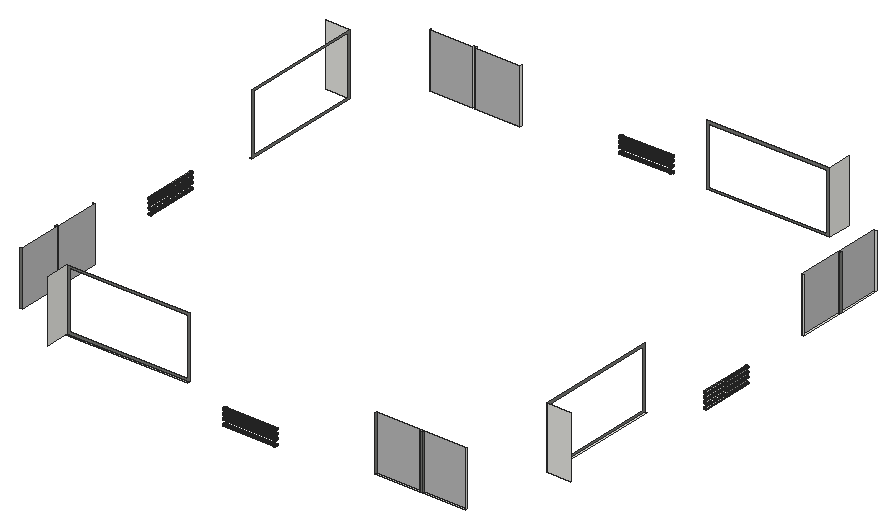
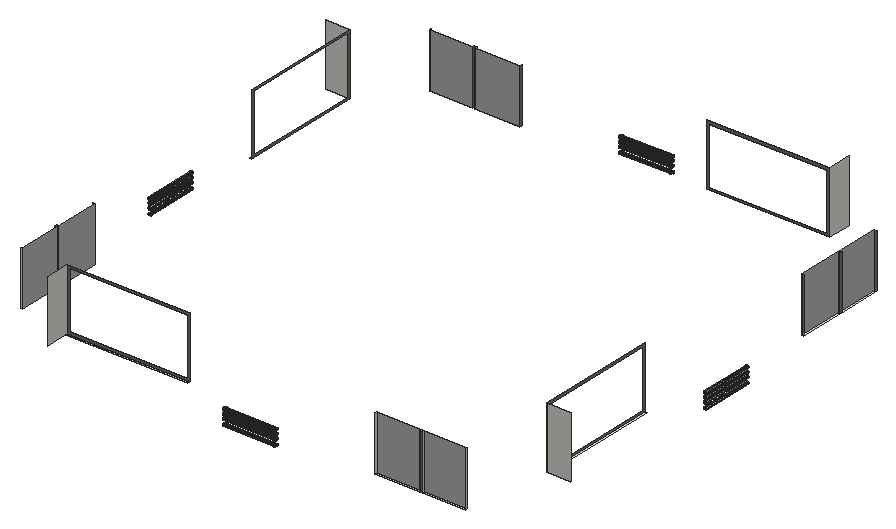
# SketchUp Ruby script. Lengths in inches.
U = 1.inch
M = Sketchup.active_model
def pt(a) = Geom::Point3d.new(a.map { |v| v * U })
def face(e, loops, mat)
  f = e.add_face(loops[0].map { |a| pt(a) })
  loops[1..].each { |l| e.add_face(l.map { |a| pt(a) }).erase! }
  f.material = f.back_material = mat if mat
  f
end
# faces: each face lists its corners as indices into pts; further lists are holes
def faces(e, pts, list, mat = nil) = list.each { |f| face(e, (f[0].is_a?(Array) ? f : [f]).map { |l| l.map { |i| pts[i] } }, mat) }
# xy, xz, yz: faces in a plane at the given z, y or x. An outline is a flat list of corners, or four numbers for a rectangle; further outlines are holes
def ring(l) = l.size == 4 ? [[l[0], l[1]], [l[2], l[1]], [l[2], l[3]], [l[0], l[3]]] : l.each_slice(2).to_a
def flat(e, list, mat, &to3) = list.each { |f| face(e, (f[0].is_a?(Array) ? f : [f]).map { |l| ring(l).map { |u, v| to3.(u, v) } }, mat) }
def xy(e, z, list, mat = nil) = flat(e, list, mat) { |x, y| [x, y, z] }
def xz(e, y, list, mat = nil) = flat(e, list, mat) { |x, z| [x, y, z] }
def yz(e, x, list, mat = nil) = flat(e, list, mat) { |y, z| [x, y, z] }
def lines(e, pts, list) = list.each { |a, b| e.add_line(pt(pts[a]), pt(pts[b])) }
# prism: a flat outline (further loops are holes) pulled along v
def prism(e, loops, v, mat = nil)
  f = face(e, loops, mat); d = Geom::Vector3d.new(v.map { |x| x * U })
  f.pushpull(f.normal.samedirection?(d) ? d.length : -d.length)
end
def box(e, o, s, mat = nil) = prism(e, [[o, [o[0] + s[0], o[1], o[2]], [o[0] + s[0], o[1] + s[1], o[2]], [o[0], o[1] + s[1], o[2]]]], [0, 0, s[2]], mat)
def at(x, y, z, deg = 0) = Geom::Transformation.translation(pt([x, y, z])) * Geom::Transformation.rotation(ORIGIN, Z_AXIS, deg.degrees)
def axes(o, x, y, z) = Geom::Transformation.new([*x, 0, *y, 0, *z, 0, *pt(o).to_a, 1])
def part(name) = M.definitions.add(name)
# library, detail: a bought-in or finely detailed component or shape, given as its bounding box
def library(name, o, s) = part(name).tap { |d| box(d.entities, o, s) }
def detail(e, o, s) = box(e.add_group.entities, o, s)
def put(e, d, t, mat = nil) = e.add_instance(d, t).tap { |i| i.material = mat if mat }
def group(e, t, mat = nil) = e.add_group.tap { |g| g.transformation = t; g.material = mat if mat }.entities
root = M.entities
M.materials.add("[Metal Seamed]").color = [118, 119, 115]
M.materials.add("[Mirror 01]").color = [185, 185, 185]
xy(root,1579.11,[[1161.2,84.8125,1285.04,90.8125],[1291.04,84.8125,1408.89,90.8125],[120,175.92,126,293.77],[120,299.77,126,423.61],[1494,1126.01,1500,1249.86],
  [1494,1255.86,1500,1373.7],[211.11,1458.8125,328.96,1464.8125],[334.96,1458.8125,458.8,1464.8125]])
xy(root,1613.76,[[306.65,96.8125,641.22,102.8125],[1482,271.47,1488,606.03],[132,943.59,138,1278.16],[978.78,1446.8125,1313.35,1452.8125]])
xz(root,84.8125,[[1285.04,1579.11,1291.04,1727.61]],"[Metal Seamed]")
xz(root,90.8125,[[1161.2,1579.11,1285.04,1727.61],[1291.04,1579.11,1408.89,1727.61]],"[Mirror 01]")
xz(root,102.8125,[[[306.65,1613.76,641.22,1782.625],[312.65,1619.76,635.22,1776.625]]],"[Metal Seamed]")
xz(root,175.92,[[120,1579.11,126,1727.61]],"[Metal Seamed]")
xz(root,271.47,[[1482,1613.76,1548,1782.625]])
xz(root,293.77,[[120,1579.11,126,1727.61]],"[Metal Seamed]")
xz(root,299.77,[[120,1579.11,126,1727.61]],"[Metal Seamed]")
xz(root,423.61,[[120,1579.11,126,1727.61]],"[Metal Seamed]")
xz(root,1126.01,[[1494,1579.11,1500,1727.61]])
xz(root,1249.86,[[1494,1579.11,1500,1727.61]])
xz(root,1255.86,[[1494,1579.11,1500,1727.61]])
xz(root,1278.16,[[72,1613.76,138,1782.625]])
xz(root,1373.7,[[1494,1579.11,1500,1727.61]])
xz(root,1446.8125,[[[978.78,1613.76,1313.35,1782.625],[984.78,1619.76,1307.35,1776.625]]],"[Metal Seamed]")
xz(root,1458.8125,[[211.11,1579.11,328.96,1727.61],[334.96,1579.11,458.8,1727.61]],"[Mirror 01]")
xz(root,1464.8125,[[328.96,1579.11,334.96,1727.61]],"[Metal Seamed]")
yz(root,120,[[293.77,1579.11,299.77,1727.61]],"[Metal Seamed]")
yz(root,126,[[175.92,1579.11,293.77,1727.61],[299.77,1579.11,423.61,1727.61]],"[Mirror 01]")
yz(root,138,[[[943.59,1613.76,1278.16,1782.625],[949.59,1619.76,1272.16,1776.625]]],"[Metal Seamed]")
yz(root,211.11,[[1458.8125,1579.11,1464.8125,1727.61]])
yz(root,306.65,[[36.8125,1613.76,102.8125,1782.625]])
yz(root,328.96,[[1458.8125,1579.11,1464.8125,1727.61]])
yz(root,334.96,[[1458.8125,1579.11,1464.8125,1727.61]])
yz(root,458.8,[[1458.8125,1579.11,1464.8125,1727.61]])
yz(root,1161.2,[[84.8125,1579.11,90.8125,1727.61]],"[Metal Seamed]")
yz(root,1285.04,[[84.8125,1579.11,90.8125,1727.61]])
yz(root,1291.04,[[84.8125,1579.11,90.8125,1727.61]],"[Metal Seamed]")
yz(root,1313.35,[[1446.8125,1613.76,1512.8125,1782.625]])
yz(root,1408.89,[[84.8125,1579.11,90.8125,1727.61]])
yz(root,1482,[[[271.47,1613.76,606.03,1782.625],[277.47,1619.76,600.03,1776.625]]],"[Metal Seamed]")
yz(root,1494,[[1126.01,1579.11,1249.86,1727.61],[1255.86,1579.11,1373.7,1727.61]],"[Mirror 01]")
yz(root,1500,[[1249.86,1579.11,1255.86,1727.61]],"[Metal Seamed]")
p = [[922.01,45.73,1579.1],[922.01,45.15,1579.86],[778.64,45.15,1579.86],[778.64,45.73,1579.1],[922.01,51.53,1579.86],[922.01,50.95,1579.1],
  [778.64,50.95,1579.1],[778.64,51.53,1579.86],[80.92,662.8,1579.1],[80.33,662.8,1579.86],[80.33,806.17,1579.86],[80.92,806.17,1579.1],
  [86.72,662.8,1579.86],[86.13,662.8,1579.1],[86.13,806.17,1579.1],[86.72,806.17,1579.86],[1533.28,886.83,1579.86],[1533.87,886.83,1579.1],
  [1533.87,743.45,1579.1],[1533.28,743.45,1579.86],[1539.08,886.83,1579.1],[1539.67,886.83,1579.86],[1539.67,743.45,1579.86],[1539.08,743.45,1579.1],
  [697.99,1498.09,1579.86],[697.99,1498.68,1579.1],[841.36,1498.68,1579.1],[841.36,1498.09,1579.86],[697.99,1503.89,1579.1],[697.99,1504.48,1579.86],
  [841.36,1504.48,1579.86],[841.36,1503.89,1579.1],[922.01,44.78,1580.75],[778.64,44.78,1580.75],[922.01,51.9,1580.75],[778.64,51.9,1580.75],
  [79.97,662.8,1580.75],[79.97,806.17,1580.75],[87.09,662.8,1580.75],[87.09,806.17,1580.75],[1532.91,886.83,1580.75],[1532.91,743.45,1580.75],
  [1540.03,886.83,1580.75],[1540.03,743.45,1580.75],[697.99,1497.72,1580.75],[841.36,1497.72,1580.75],[697.99,1504.85,1580.75],[841.36,1504.85,1580.75],
  [922.01,44.65,1581.7],[778.64,44.65,1581.7],[922.01,52.03,1581.7],[778.64,52.03,1581.7],[79.84,662.8,1581.7],[79.84,806.17,1581.7],
  [87.21,662.8,1581.7],[87.21,806.17,1581.7],[1532.79,886.83,1581.7],[1532.79,743.45,1581.7],[1540.16,886.83,1581.7],[1540.16,743.45,1581.7],
  [697.99,1497.6,1581.7],[841.36,1497.6,1581.7],[697.99,1504.97,1581.7],[841.36,1504.97,1581.7],[922.01,44.78,1582.66],[778.64,44.78,1582.66],
  [922.01,51.9,1582.66],[778.64,51.9,1582.66],[79.97,662.8,1582.66],[79.97,806.17,1582.66],[87.09,662.8,1582.66],[87.09,806.17,1582.66],
  [1532.91,886.83,1582.66],[1532.91,743.45,1582.66],[1540.03,886.83,1582.66],[1540.03,743.45,1582.66],[697.99,1497.72,1582.66],[841.36,1497.72,1582.66],
  [697.99,1504.85,1582.66],[841.36,1504.85,1582.66],[922.01,45.15,1583.55],[778.64,45.15,1583.55],[922.01,51.53,1583.55],[778.64,51.53,1583.55],
  [80.33,662.8,1583.55],[80.33,806.17,1583.55],[86.72,662.8,1583.55],[86.72,806.17,1583.55],[1533.28,886.83,1583.55],[1533.28,743.45,1583.55],
  [1539.67,886.83,1583.55],[1539.67,743.45,1583.55],[697.99,1498.09,1583.55],[841.36,1498.09,1583.55],[697.99,1504.48,1583.55],[841.36,1504.48,1583.55],
  [922.01,45.73,1584.3125],[778.64,45.73,1584.3125],[922.01,50.95,1584.3125],[778.64,50.95,1584.3125],[80.92,662.8,1584.3125],[80.92,806.17,1584.3125],
  [86.13,662.8,1584.3125],[86.13,806.17,1584.3125],[1533.87,886.83,1584.3125],[1533.87,743.45,1584.3125],[1539.08,886.83,1584.3125],[1539.08,743.45,1584.3125],
  [697.99,1498.68,1584.3125],[841.36,1498.68,1584.3125],[697.99,1503.89,1584.3125],[841.36,1503.89,1584.3125],[922.01,46.5,1584.9],[778.64,46.5,1584.9],
  [922.01,50.18,1584.9],[778.64,50.18,1584.9],[81.68,662.8,1584.9],[81.68,806.17,1584.9],[85.37,662.8,1584.9],[85.37,806.17,1584.9],
  [1534.63,886.83,1584.9],[1534.63,743.45,1584.9],[1538.32,886.83,1584.9],[1538.32,743.45,1584.9],[697.99,1499.44,1584.9],[841.36,1499.44,1584.9],
  [697.99,1503.13,1584.9],[841.36,1503.13,1584.9],[922.01,47.38,1585.27],[778.64,47.38,1585.27],[922.01,49.29,1585.27],[778.64,49.29,1585.27],
  [82.57,662.8,1585.27],[82.57,806.17,1585.27],[84.48,662.8,1585.27],[84.48,806.17,1585.27],[1535.52,886.83,1585.27],[1535.52,743.45,1585.27],
  [1537.43,886.83,1585.27],[1537.43,743.45,1585.27],[697.99,1500.33,1585.27],[841.36,1500.33,1585.27],[697.99,1502.24,1585.27],[841.36,1502.24,1585.27],
  [922.01,48.34,1585.39],[778.64,48.34,1585.39],[83.53,662.8,1585.39],[83.53,806.17,1585.39],[1536.47,886.83,1585.39],[1536.47,743.45,1585.39],
  [697.99,1501.28,1585.39],[841.36,1501.28,1585.39],[922.01,48.34,1593.02],[922.01,47.38,1593.14],[778.64,47.38,1593.14],[778.64,48.34,1593.02],
  [922.01,49.29,1593.14],[778.64,49.29,1593.14],[83.53,662.8,1593.02],[82.57,662.8,1593.14],[82.57,806.17,1593.14],[83.53,806.17,1593.02],
  [84.48,662.8,1593.14],[84.48,806.17,1593.14],[1535.52,886.83,1593.14],[1536.47,886.83,1593.02],[1536.47,743.45,1593.02],[1535.52,743.45,1593.14],
  [1537.43,886.83,1593.14],[1537.43,743.45,1593.14],[697.99,1500.33,1593.14],[697.99,1501.28,1593.02],[841.36,1501.28,1593.02],[841.36,1500.33,1593.14],
  [697.99,1502.24,1593.14],[841.36,1502.24,1593.14],[922.01,46.5,1593.51],[778.64,46.5,1593.51],[922.01,50.18,1593.51],[778.64,50.18,1593.51],
  [81.68,662.8,1593.51],[81.68,806.17,1593.51],[85.37,662.8,1593.51],[85.37,806.17,1593.51],[1534.63,886.83,1593.51],[1534.63,743.45,1593.51],
  [1538.32,886.83,1593.51],[1538.32,743.45,1593.51],[697.99,1499.44,1593.51],[841.36,1499.44,1593.51],[697.99,1503.13,1593.51],[841.36,1503.13,1593.51],
  [922.01,45.73,1594.1],[778.64,45.73,1594.1],[922.01,50.95,1594.1],[778.64,50.95,1594.1],[80.92,662.8,1594.1],[80.92,806.17,1594.1],
  [86.13,662.8,1594.1],[86.13,806.17,1594.1],[1533.87,886.83,1594.1],[1533.87,743.45,1594.1],[1539.08,886.83,1594.1],[1539.08,743.45,1594.1],
  [697.99,1498.68,1594.1],[841.36,1498.68,1594.1],[697.99,1503.89,1594.1],[841.36,1503.89,1594.1],[922.01,45.15,1594.86],[778.64,45.15,1594.86],
  [922.01,51.53,1594.86],[778.64,51.53,1594.86],[80.33,662.8,1594.86],[80.33,806.17,1594.86],[86.72,662.8,1594.86],[86.72,806.17,1594.86],
  [1533.28,886.83,1594.86],[1533.28,743.45,1594.86],[1539.67,886.83,1594.86],[1539.67,743.45,1594.86],[697.99,1498.09,1594.86],[841.36,1498.09,1594.86],
  [697.99,1504.48,1594.86],[841.36,1504.48,1594.86],[922.01,44.78,1595.75],[778.64,44.78,1595.75],[922.01,51.9,1595.75],[778.64,51.9,1595.75],
  [79.97,662.8,1595.75],[79.97,806.17,1595.75],[87.09,662.8,1595.75],[87.09,806.17,1595.75],[1532.91,886.83,1595.75],[1532.91,743.45,1595.75],
  [1540.03,886.83,1595.75],[1540.03,743.45,1595.75],[697.99,1497.72,1595.75],[841.36,1497.72,1595.75],[697.99,1504.85,1595.75],[841.36,1504.85,1595.75],
  [922.01,44.65,1596.7],[778.64,44.65,1596.7],[922.01,52.03,1596.7],[778.64,52.03,1596.7],[79.84,662.8,1596.7],[79.84,806.17,1596.7],
  [87.21,662.8,1596.7],[87.21,806.17,1596.7],[1532.79,886.83,1596.7],[1532.79,743.45,1596.7],[1540.16,886.83,1596.7],[1540.16,743.45,1596.7],
  [697.99,1497.6,1596.7],[841.36,1497.6,1596.7],[697.99,1504.97,1596.7],[841.36,1504.97,1596.7],[922.01,44.78,1597.66],[778.64,44.78,1597.66],
  [922.01,51.9,1597.66],[778.64,51.9,1597.66],[79.97,662.8,1597.66],[79.97,806.17,1597.66],[87.09,662.8,1597.66],[87.09,806.17,1597.66],
  [1532.91,886.83,1597.66],[1532.91,743.45,1597.66],[1540.03,886.83,1597.66],[1540.03,743.45,1597.66],[697.99,1497.72,1597.66],[841.36,1497.72,1597.66],
  [697.99,1504.85,1597.66],[841.36,1504.85,1597.66],[922.01,45.15,1598.55],[778.64,45.15,1598.55],[922.01,51.53,1598.55],[778.64,51.53,1598.55],
  [80.33,662.8,1598.55],[80.33,806.17,1598.55],[86.72,662.8,1598.55],[86.72,806.17,1598.55],[1533.28,886.83,1598.55],[1533.28,743.45,1598.55],
  [1539.67,886.83,1598.55],[1539.67,743.45,1598.55],[697.99,1498.09,1598.55],[841.36,1498.09,1598.55],[697.99,1504.48,1598.55],[841.36,1504.48,1598.55],
  [922.01,45.73,1599.3125],[778.64,45.73,1599.3125],[922.01,50.95,1599.3125],[778.64,50.95,1599.3125],[80.92,662.8,1599.3125],[80.92,806.17,1599.3125],
  [86.13,662.8,1599.3125],[86.13,806.17,1599.3125],[1533.87,886.83,1599.3125],[1533.87,743.45,1599.3125],[1539.08,886.83,1599.3125],[1539.08,743.45,1599.3125],
  [697.99,1498.68,1599.3125],[841.36,1498.68,1599.3125],[697.99,1503.89,1599.3125],[841.36,1503.89,1599.3125],[922.01,46.5,1599.9],[778.64,46.5,1599.9],
  [922.01,50.18,1599.9],[778.64,50.18,1599.9],[81.68,662.8,1599.9],[81.68,806.17,1599.9],[85.37,662.8,1599.9],[85.37,806.17,1599.9],
  [1534.63,886.83,1599.9],[1534.63,743.45,1599.9],[1538.32,886.83,1599.9],[1538.32,743.45,1599.9],[697.99,1499.44,1599.9],[841.36,1499.44,1599.9],
  [697.99,1503.13,1599.9],[841.36,1503.13,1599.9],[922.01,47.38,1600.27],[778.64,47.38,1600.27],[922.01,49.29,1600.27],[778.64,49.29,1600.27],
  [82.57,662.8,1600.27],[82.57,806.17,1600.27],[84.48,662.8,1600.27],[84.48,806.17,1600.27],[1535.52,886.83,1600.27],[1535.52,743.45,1600.27],
  [1537.43,886.83,1600.27],[1537.43,743.45,1600.27],[697.99,1500.33,1600.27],[841.36,1500.33,1600.27],[697.99,1502.24,1600.27],[841.36,1502.24,1600.27],
  [922.01,48.34,1600.39],[778.64,48.34,1600.39],[83.53,662.8,1600.39],[83.53,806.17,1600.39],[1536.47,886.83,1600.39],[1536.47,743.45,1600.39],
  [697.99,1501.28,1600.39],[841.36,1501.28,1600.39],[922.01,48.34,1605.02],[922.01,47.38,1605.14],[778.64,47.38,1605.14],[778.64,48.34,1605.02],
  [922.01,49.29,1605.14],[778.64,49.29,1605.14],[83.53,662.8,1605.02],[82.57,662.8,1605.14],[82.57,806.17,1605.14],[83.53,806.17,1605.02],
  [84.48,662.8,1605.14],[84.48,806.17,1605.14],[1535.52,886.83,1605.14],[1536.47,886.83,1605.02],[1536.47,743.45,1605.02],[1535.52,743.45,1605.14],
  [1537.43,886.83,1605.14],[1537.43,743.45,1605.14],[697.99,1500.33,1605.14],[697.99,1501.28,1605.02],[841.36,1501.28,1605.02],[841.36,1500.33,1605.14],
  [697.99,1502.24,1605.14],[841.36,1502.24,1605.14],[922.01,46.5,1605.51],[778.64,46.5,1605.51],[922.01,50.18,1605.51],[778.64,50.18,1605.51],
  [81.68,662.8,1605.51],[81.68,806.17,1605.51],[85.37,662.8,1605.51],[85.37,806.17,1605.51],[1534.63,886.83,1605.51],[1534.63,743.45,1605.51],
  [1538.32,886.83,1605.51],[1538.32,743.45,1605.51],[697.99,1499.44,1605.51],[841.36,1499.44,1605.51],[697.99,1503.13,1605.51],[841.36,1503.13,1605.51],
  [922.01,45.73,1606.1],[778.64,45.73,1606.1],[922.01,50.95,1606.1],[778.64,50.95,1606.1],[80.92,662.8,1606.1],[80.92,806.17,1606.1],
  [86.13,662.8,1606.1],[86.13,806.17,1606.1],[1533.87,886.83,1606.1],[1533.87,743.45,1606.1],[1539.08,886.83,1606.1],[1539.08,743.45,1606.1],
  [697.99,1498.68,1606.1],[841.36,1498.68,1606.1],[697.99,1503.89,1606.1],[841.36,1503.89,1606.1],[922.01,45.15,1606.86],[778.64,45.15,1606.86],
  [922.01,51.53,1606.86],[778.64,51.53,1606.86],[80.33,662.8,1606.86],[80.33,806.17,1606.86],[86.72,662.8,1606.86],[86.72,806.17,1606.86],
  [1533.28,886.83,1606.86],[1533.28,743.45,1606.86],[1539.67,886.83,1606.86],[1539.67,743.45,1606.86],[697.99,1498.09,1606.86],[841.36,1498.09,1606.86],
  [697.99,1504.48,1606.86],[841.36,1504.48,1606.86],[922.01,44.78,1607.75],[778.64,44.78,1607.75],[922.01,51.9,1607.75],[778.64,51.9,1607.75],
  [79.97,662.8,1607.75],[79.97,806.17,1607.75],[87.09,662.8,1607.75],[87.09,806.17,1607.75],[1532.91,886.83,1607.75],[1532.91,743.45,1607.75],
  [1540.03,886.83,1607.75],[1540.03,743.45,1607.75],[697.99,1497.72,1607.75],[841.36,1497.72,1607.75],[697.99,1504.85,1607.75],[841.36,1504.85,1607.75],
  [922.01,44.65,1608.7],[778.64,44.65,1608.7],[922.01,52.03,1608.7],[778.64,52.03,1608.7],[79.84,662.8,1608.7],[79.84,806.17,1608.7],
  [87.21,662.8,1608.7],[87.21,806.17,1608.7],[1532.79,886.83,1608.7],[1532.79,743.45,1608.7],[1540.16,886.83,1608.7],[1540.16,743.45,1608.7],
  [697.99,1497.6,1608.7],[841.36,1497.6,1608.7],[697.99,1504.97,1608.7],[841.36,1504.97,1608.7],[922.01,44.78,1609.66],[778.64,44.78,1609.66],
  [922.01,51.9,1609.66],[778.64,51.9,1609.66],[79.97,662.8,1609.66],[79.97,806.17,1609.66],[87.09,662.8,1609.66],[87.09,806.17,1609.66],
  [1532.91,886.83,1609.66],[1532.91,743.45,1609.66],[1540.03,886.83,1609.66],[1540.03,743.45,1609.66],[697.99,1497.72,1609.66],[841.36,1497.72,1609.66],
  [697.99,1504.85,1609.66],[841.36,1504.85,1609.66],[922.01,45.15,1610.55],[778.64,45.15,1610.55],[922.01,51.53,1610.55],[778.64,51.53,1610.55],
  [80.33,662.8,1610.55],[80.33,806.17,1610.55],[86.72,662.8,1610.55],[86.72,806.17,1610.55],[1533.28,886.83,1610.55],[1533.28,743.45,1610.55],
  [1539.67,886.83,1610.55],[1539.67,743.45,1610.55],[697.99,1498.09,1610.55],[841.36,1498.09,1610.55],[697.99,1504.48,1610.55],[841.36,1504.48,1610.55],
  [922.01,45.73,1611.3125],[778.64,45.73,1611.3125],[922.01,50.95,1611.3125],[778.64,50.95,1611.3125],[80.92,662.8,1611.3125],[80.92,806.17,1611.3125],
  [86.13,662.8,1611.3125],[86.13,806.17,1611.3125],[1533.87,886.83,1611.3125],[1533.87,743.45,1611.3125],[1539.08,886.83,1611.3125],[1539.08,743.45,1611.3125],
  [697.99,1498.68,1611.3125],[841.36,1498.68,1611.3125],[697.99,1503.89,1611.3125],[841.36,1503.89,1611.3125],[922.01,46.5,1611.9],[778.64,46.5,1611.9],
  [922.01,50.18,1611.9],[778.64,50.18,1611.9],[81.68,662.8,1611.9],[81.68,806.17,1611.9],[85.37,662.8,1611.9],[85.37,806.17,1611.9],
  [1534.63,886.83,1611.9],[1534.63,743.45,1611.9],[1538.32,886.83,1611.9],[1538.32,743.45,1611.9],[697.99,1499.44,1611.9],[841.36,1499.44,1611.9],
  [697.99,1503.13,1611.9],[841.36,1503.13,1611.9],[922.01,47.38,1612.27],[778.64,47.38,1612.27],[922.01,49.29,1612.27],[778.64,49.29,1612.27],
  [82.57,662.8,1612.27],[82.57,806.17,1612.27],[84.48,662.8,1612.27],[84.48,806.17,1612.27],[1535.52,886.83,1612.27],[1535.52,743.45,1612.27],
  [1537.43,886.83,1612.27],[1537.43,743.45,1612.27],[697.99,1500.33,1612.27],[841.36,1500.33,1612.27],[697.99,1502.24,1612.27],[841.36,1502.24,1612.27],
  [922.01,48.34,1612.39],[778.64,48.34,1612.39],[83.53,662.8,1612.39],[83.53,806.17,1612.39],[1536.47,886.83,1612.39],[1536.47,743.45,1612.39],
  [697.99,1501.28,1612.39],[841.36,1501.28,1612.39],[922.01,48.34,1617.02],[922.01,47.38,1617.14],[778.64,47.38,1617.14],[778.64,48.34,1617.02],
  [922.01,49.29,1617.14],[778.64,49.29,1617.14],[83.53,662.8,1617.02],[82.57,662.8,1617.14],[82.57,806.17,1617.14],[83.53,806.17,1617.02],
  [84.48,662.8,1617.14],[84.48,806.17,1617.14],[1535.52,886.83,1617.14],[1536.47,886.83,1617.02],[1536.47,743.45,1617.02],[1535.52,743.45,1617.14],
  [1537.43,886.83,1617.14],[1537.43,743.45,1617.14],[697.99,1500.33,1617.14],[697.99,1501.28,1617.02],[841.36,1501.28,1617.02],[841.36,1500.33,1617.14],
  [697.99,1502.24,1617.14],[841.36,1502.24,1617.14],[922.01,46.5,1617.51],[778.64,46.5,1617.51],[922.01,50.18,1617.51],[778.64,50.18,1617.51],
  [81.68,662.8,1617.51],[81.68,806.17,1617.51],[85.37,662.8,1617.51],[85.37,806.17,1617.51],[1534.63,886.83,1617.51],[1534.63,743.45,1617.51],
  [1538.32,886.83,1617.51],[1538.32,743.45,1617.51],[697.99,1499.44,1617.51],[841.36,1499.44,1617.51],[697.99,1503.13,1617.51],[841.36,1503.13,1617.51],
  [922.01,45.73,1618.1],[778.64,45.73,1618.1],[922.01,50.95,1618.1],[778.64,50.95,1618.1],[80.92,662.8,1618.1],[80.92,806.17,1618.1],
  [86.13,662.8,1618.1],[86.13,806.17,1618.1],[1533.87,886.83,1618.1],[1533.87,743.45,1618.1],[1539.08,886.83,1618.1],[1539.08,743.45,1618.1],
  [697.99,1498.68,1618.1],[841.36,1498.68,1618.1],[697.99,1503.89,1618.1],[841.36,1503.89,1618.1],[922.01,45.15,1618.86],[778.64,45.15,1618.86],
  [922.01,51.53,1618.86],[778.64,51.53,1618.86],[80.33,662.8,1618.86],[80.33,806.17,1618.86],[86.72,662.8,1618.86],[86.72,806.17,1618.86],
  [1533.28,886.83,1618.86],[1533.28,743.45,1618.86],[1539.67,886.83,1618.86],[1539.67,743.45,1618.86],[697.99,1498.09,1618.86],[841.36,1498.09,1618.86],
  [697.99,1504.48,1618.86],[841.36,1504.48,1618.86],[922.01,44.78,1619.75],[778.64,44.78,1619.75],[922.01,51.9,1619.75],[778.64,51.9,1619.75],
  [79.97,662.8,1619.75],[79.97,806.17,1619.75],[87.09,662.8,1619.75],[87.09,806.17,1619.75],[1532.91,886.83,1619.75],[1532.91,743.45,1619.75],
  [1540.03,886.83,1619.75],[1540.03,743.45,1619.75],[697.99,1497.72,1619.75],[841.36,1497.72,1619.75],[697.99,1504.85,1619.75],[841.36,1504.85,1619.75],
  [922.01,44.65,1620.7],[778.64,44.65,1620.7],[922.01,52.03,1620.7],[778.64,52.03,1620.7],[79.84,662.8,1620.7],[79.84,806.17,1620.7],
  [87.21,662.8,1620.7],[87.21,806.17,1620.7],[1532.79,886.83,1620.7],[1532.79,743.45,1620.7],[1540.16,886.83,1620.7],[1540.16,743.45,1620.7],
  [697.99,1497.6,1620.7],[841.36,1497.6,1620.7],[697.99,1504.97,1620.7],[841.36,1504.97,1620.7],[922.01,44.78,1621.66],[778.64,44.78,1621.66],
  [922.01,51.9,1621.66],[778.64,51.9,1621.66],[79.97,662.8,1621.66],[79.97,806.17,1621.66],[87.09,662.8,1621.66],[87.09,806.17,1621.66],
  [1532.91,886.83,1621.66],[1532.91,743.45,1621.66],[1540.03,886.83,1621.66],[1540.03,743.45,1621.66],[697.99,1497.72,1621.66],[841.36,1497.72,1621.66],
  [697.99,1504.85,1621.66],[841.36,1504.85,1621.66],[922.01,45.15,1622.55],[778.64,45.15,1622.55],[922.01,51.53,1622.55],[778.64,51.53,1622.55],
  [80.33,662.8,1622.55],[80.33,806.17,1622.55],[86.72,662.8,1622.55],[86.72,806.17,1622.55],[1533.28,886.83,1622.55],[1533.28,743.45,1622.55],
  [1539.67,886.83,1622.55],[1539.67,743.45,1622.55],[697.99,1498.09,1622.55],[841.36,1498.09,1622.55],[697.99,1504.48,1622.55],[841.36,1504.48,1622.55],
  [922.01,45.73,1623.3125],[778.64,45.73,1623.3125],[922.01,50.95,1623.3125],[778.64,50.95,1623.3125],[80.92,662.8,1623.3125],[80.92,806.17,1623.3125],
  [86.13,662.8,1623.3125],[86.13,806.17,1623.3125],[1533.87,886.83,1623.3125],[1533.87,743.45,1623.3125],[1539.08,886.83,1623.3125],[1539.08,743.45,1623.3125],
  [697.99,1498.68,1623.3125],[841.36,1498.68,1623.3125],[697.99,1503.89,1623.3125],[841.36,1503.89,1623.3125],[922.01,46.5,1623.9],[778.64,46.5,1623.9],
  [922.01,50.18,1623.9],[778.64,50.18,1623.9],[81.68,662.8,1623.9],[81.68,806.17,1623.9],[85.37,662.8,1623.9],[85.37,806.17,1623.9],
  [1534.63,886.83,1623.9],[1534.63,743.45,1623.9],[1538.32,886.83,1623.9],[1538.32,743.45,1623.9],[697.99,1499.44,1623.9],[841.36,1499.44,1623.9],
  [697.99,1503.13,1623.9],[841.36,1503.13,1623.9],[922.01,47.38,1624.27],[778.64,47.38,1624.27],[922.01,49.29,1624.27],[778.64,49.29,1624.27],
  [82.57,662.8,1624.27],[82.57,806.17,1624.27],[84.48,662.8,1624.27],[84.48,806.17,1624.27],[1535.52,886.83,1624.27],[1535.52,743.45,1624.27],
  [1537.43,886.83,1624.27],[1537.43,743.45,1624.27],[697.99,1500.33,1624.27],[841.36,1500.33,1624.27],[697.99,1502.24,1624.27],[841.36,1502.24,1624.27],
  [922.01,48.34,1624.39],[778.64,48.34,1624.39],[83.53,662.8,1624.39],[83.53,806.17,1624.39],[1536.47,886.83,1624.39],[1536.47,743.45,1624.39],
  [697.99,1501.28,1624.39],[841.36,1501.28,1624.39],[922.01,48.34,1581.7],[778.64,48.34,1581.7],[697.99,1501.28,1581.7],[841.36,1501.28,1581.7],
  [83.53,662.8,1581.7],[83.53,806.17,1581.7],[1536.47,886.83,1581.7],[1536.47,743.45,1581.7]]
faces(root,p,[[0,1,2,3],[4,5,6,7],[8,9,10,11],[12,13,14,15],[16,17,18,19],[20,21,22,23],[24,25,26,27],[28,29,30,31],
  [1,32,33,2],[34,4,7,35],[9,36,37,10],[38,12,15,39],[40,16,19,41],[21,42,43,22],[44,24,27,45],[29,46,47,30],
  [32,48,49,33],[50,34,35,51],[36,52,53,37],[54,38,39,55],[56,40,41,57],[42,58,59,43],[60,44,45,61],[46,62,63,47],
  [48,64,65,49],[66,50,51,67],[52,68,69,53],[70,54,55,71],[72,56,57,73],[58,74,75,59],[76,60,61,77],[62,78,79,63],
  [64,80,81,65],[82,66,67,83],[68,84,85,69],[86,70,71,87],[88,72,73,89],[74,90,91,75],[92,76,77,93],[78,94,95,79],
  [80,96,97,81],[98,82,83,99],[84,100,101,85],[102,86,87,103],[104,88,89,105],[90,106,107,91],[108,92,93,109],[94,110,111,95],
  [96,112,113,97],[114,98,99,115],[100,116,117,101],[118,102,103,119],[120,104,105,121],[106,122,123,107],[124,108,109,125],[110,126,127,111],
  [112,128,129,113],[130,114,115,131],[116,132,133,117],[134,118,119,135],[136,120,121,137],[122,138,139,123],[140,124,125,141],[126,142,143,127],
  [128,144,145,129],[144,130,131,145],[132,146,147,133],[146,134,135,147],[148,136,137,149],[138,148,149,139],[150,140,141,151],[142,150,151,143],
  [152,153,154,155],[156,152,155,157],[158,159,160,161],[162,158,161,163],[164,165,166,167],[165,168,169,166],[170,171,172,173],[171,174,175,172],
  [153,176,177,154],[178,156,157,179],[159,180,181,160],[182,162,163,183],[184,164,167,185],[168,186,187,169],[188,170,173,189],[174,190,191,175],
  [176,192,193,177],[194,178,179,195],[180,196,197,181],[198,182,183,199],[200,184,185,201],[186,202,203,187],[204,188,189,205],[190,206,207,191],
  [192,208,209,193],[210,194,195,211],[196,212,213,197],[214,198,199,215],[216,200,201,217],[202,218,219,203],[220,204,205,221],[206,222,223,207],
  [208,224,225,209],[226,210,211,227],[212,228,229,213],[230,214,215,231],[232,216,217,233],[218,234,235,219],[236,220,221,237],[222,238,239,223],
  [224,240,241,225],[242,226,227,243],[228,244,245,229],[246,230,231,247],[248,232,233,249],[234,250,251,235],[252,236,237,253],[238,254,255,239],
  [240,256,257,241],[258,242,243,259],[244,260,261,245],[262,246,247,263],[264,248,249,265],[250,266,267,251],[268,252,253,269],[254,270,271,255],
  [256,272,273,257],[274,258,259,275],[260,276,277,261],[278,262,263,279],[280,264,265,281],[266,282,283,267],[284,268,269,285],[270,286,287,271],
  [272,288,289,273],[290,274,275,291],[276,292,293,277],[294,278,279,295],[296,280,281,297],[282,298,299,283],[300,284,285,301],[286,302,303,287],
  [288,304,305,289],[306,290,291,307],[292,308,309,293],[310,294,295,311],[312,296,297,313],[298,314,315,299],[316,300,301,317],[302,318,319,303],
  [304,320,321,305],[322,306,307,323],[308,324,325,309],[326,310,311,327],[328,312,313,329],[314,330,331,315],[332,316,317,333],[318,334,335,319],
  [320,336,337,321],[336,322,323,337],[324,338,339,325],[338,326,327,339],[340,328,329,341],[330,340,341,331],[342,332,333,343],[334,342,343,335],
  [344,345,346,347],[348,344,347,349],[350,351,352,353],[354,350,353,355],[356,357,358,359],[357,360,361,358],[362,363,364,365],[363,366,367,364],
  [345,368,369,346],[370,348,349,371],[351,372,373,352],[374,354,355,375],[376,356,359,377],[360,378,379,361],[380,362,365,381],[366,382,383,367],
  [368,384,385,369],[386,370,371,387],[372,388,389,373],[390,374,375,391],[392,376,377,393],[378,394,395,379],[396,380,381,397],[382,398,399,383],
  [384,400,401,385],[402,386,387,403],[388,404,405,389],[406,390,391,407],[408,392,393,409],[394,410,411,395],[412,396,397,413],[398,414,415,399],
  [400,416,417,401],[418,402,403,419],[404,420,421,405],[422,406,407,423],[424,408,409,425],[410,426,427,411],[428,412,413,429],[414,430,431,415],
  [416,432,433,417],[434,418,419,435],[420,436,437,421],[438,422,423,439],[440,424,425,441],[426,442,443,427],[444,428,429,445],[430,446,447,431],
  [432,448,449,433],[450,434,435,451],[436,452,453,437],[454,438,439,455],[456,440,441,457],[442,458,459,443],[460,444,445,461],[446,462,463,447],
  [448,464,465,449],[466,450,451,467],[452,468,469,453],[470,454,455,471],[472,456,457,473],[458,474,475,459],[476,460,461,477],[462,478,479,463],
  [464,480,481,465],[482,466,467,483],[468,484,485,469],[486,470,471,487],[488,472,473,489],[474,490,491,475],[492,476,477,493],[478,494,495,479],
  [480,496,497,481],[498,482,483,499],[484,500,501,485],[502,486,487,503],[504,488,489,505],[490,506,507,491],[508,492,493,509],[494,510,511,495],
  [496,512,513,497],[514,498,499,515],[500,516,517,501],[518,502,503,519],[520,504,505,521],[506,522,523,507],[524,508,509,525],[510,526,527,511],
  [512,528,529,513],[528,514,515,529],[516,530,531,517],[530,518,519,531],[532,520,521,533],[522,532,533,523],[534,524,525,535],[526,534,535,527],
  [536,537,538,539],[540,536,539,541],[542,543,544,545],[546,542,545,547],[548,549,550,551],[549,552,553,550],[554,555,556,557],[555,558,559,556],
  [537,560,561,538],[562,540,541,563],[543,564,565,544],[566,546,547,567],[568,548,551,569],[552,570,571,553],[572,554,557,573],[558,574,575,559],
  [560,576,577,561],[578,562,563,579],[564,580,581,565],[582,566,567,583],[584,568,569,585],[570,586,587,571],[588,572,573,589],[574,590,591,575],
  [576,592,593,577],[594,578,579,595],[580,596,597,581],[598,582,583,599],[600,584,585,601],[586,602,603,587],[604,588,589,605],[590,606,607,591],
  [592,608,609,593],[610,594,595,611],[596,612,613,597],[614,598,599,615],[616,600,601,617],[602,618,619,603],[620,604,605,621],[606,622,623,607],
  [608,624,625,609],[626,610,611,627],[612,628,629,613],[630,614,615,631],[632,616,617,633],[618,634,635,619],[636,620,621,637],[622,638,639,623],
  [624,640,641,625],[642,626,627,643],[628,644,645,629],[646,630,631,647],[648,632,633,649],[634,650,651,635],[652,636,637,653],[638,654,655,639],
  [640,656,657,641],[658,642,643,659],[644,660,661,645],[662,646,647,663],[664,648,649,665],[650,666,667,651],[668,652,653,669],[654,670,671,655],
  [656,672,673,657],[674,658,659,675],[660,676,677,661],[678,662,663,679],[680,664,665,681],[666,682,683,667],[684,668,669,685],[670,686,687,671],
  [672,688,689,673],[690,674,675,691],[676,692,693,677],[694,678,679,695],[696,680,681,697],[682,698,699,683],[700,684,685,701],[686,702,703,687],
  [688,704,705,689],[706,690,691,707],[692,708,709,693],[710,694,695,711],[712,696,697,713],[698,714,715,699],[716,700,701,717],[702,718,719,703],
  [704,720,721,705],[720,706,707,721],[708,722,723,709],[722,710,711,723],[724,712,713,725],[714,724,725,715],[726,716,717,727],[718,726,727,719]])
lines(root,p,[[728,729],[730,731],[732,733],[734,735]])
